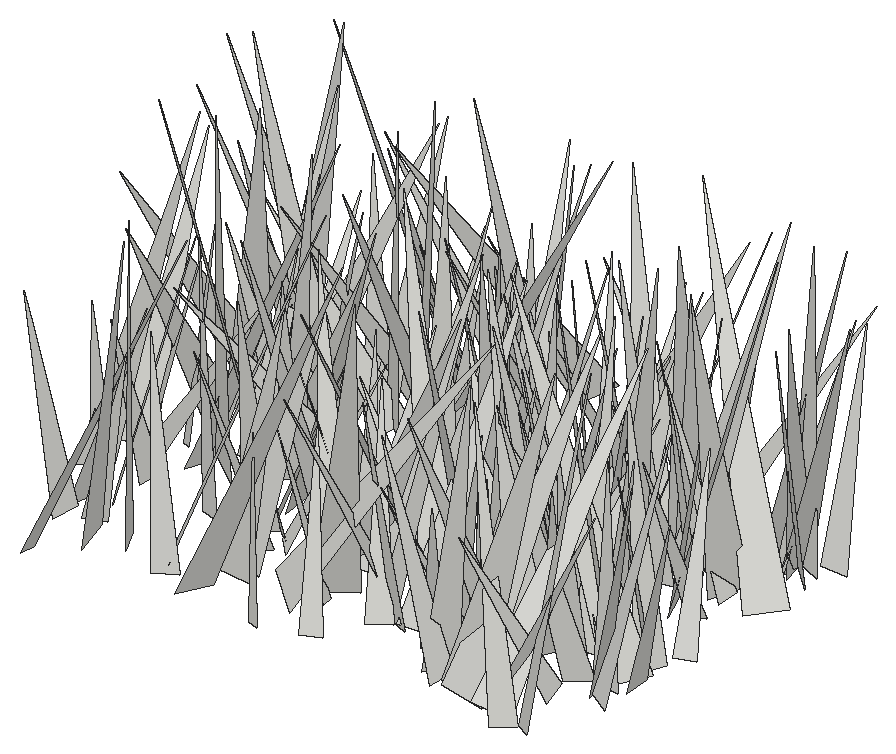
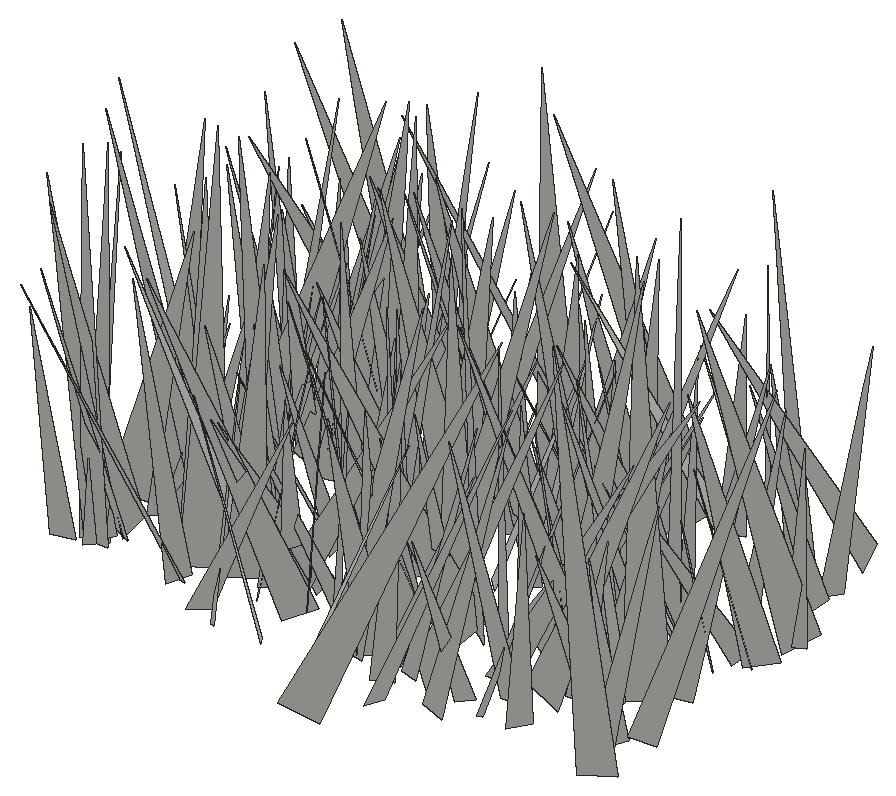
# SketchUp Ruby script. Lengths in inches.
U = 1.inch
M = Sketchup.active_model
def pt(a) = Geom::Point3d.new(a.map { |v| v * U })
def face(e, loops, mat)
  f = e.add_face(loops[0].map { |a| pt(a) })
  loops[1..].each { |l| e.add_face(l.map { |a| pt(a) }).erase! }
  f.material = f.back_material = mat if mat
  f
end
# faces: each face lists its corners as indices into pts; further lists are holes
def faces(e, pts, list, mat = nil) = list.each { |f| face(e, (f[0].is_a?(Array) ? f : [f]).map { |l| l.map { |i| pts[i] } }, mat) }
# xy, xz, yz: faces in a plane at the given z, y or x. An outline is a flat list of corners, or four numbers for a rectangle; further outlines are holes
def ring(l) = l.size == 4 ? [[l[0], l[1]], [l[2], l[1]], [l[2], l[3]], [l[0], l[3]]] : l.each_slice(2).to_a
def flat(e, list, mat, &to3) = list.each { |f| face(e, (f[0].is_a?(Array) ? f : [f]).map { |l| ring(l).map { |u, v| to3.(u, v) } }, mat) }
def xy(e, z, list, mat = nil) = flat(e, list, mat) { |x, y| [x, y, z] }
def xz(e, y, list, mat = nil) = flat(e, list, mat) { |x, z| [x, y, z] }
def yz(e, x, list, mat = nil) = flat(e, list, mat) { |y, z| [x, y, z] }
def lines(e, pts, list) = list.each { |a, b| e.add_line(pt(pts[a]), pt(pts[b])) }
# prism: a flat outline (further loops are holes) pulled along v
def prism(e, loops, v, mat = nil)
  f = face(e, loops, mat); d = Geom::Vector3d.new(v.map { |x| x * U })
  f.pushpull(f.normal.samedirection?(d) ? d.length : -d.length)
end
def box(e, o, s, mat = nil) = prism(e, [[o, [o[0] + s[0], o[1], o[2]], [o[0] + s[0], o[1] + s[1], o[2]], [o[0], o[1] + s[1], o[2]]]], [0, 0, s[2]], mat)
def at(x, y, z, deg = 0) = Geom::Transformation.translation(pt([x, y, z])) * Geom::Transformation.rotation(ORIGIN, Z_AXIS, deg.degrees)
def axes(o, x, y, z) = Geom::Transformation.new([*x, 0, *y, 0, *z, 0, *pt(o).to_a, 1])
def part(name) = M.definitions.add(name)
# library, detail: a bought-in or finely detailed component or shape, given as its bounding box
def library(name, o, s) = part(name).tap { |d| box(d.entities, o, s) }
def detail(e, o, s) = box(e.add_group.entities, o, s)
def put(e, d, t, mat = nil) = e.add_instance(d, t).tap { |i| i.material = mat if mat }
def group(e, t, mat = nil) = e.add_group.tap { |g| g.transformation = t; g.material = mat if mat }.entities
root = M.entities
c1 = part("fur_instance\#9")
p = [[0.8125,0,1.79],[0.67,-0.02,1.48],[0,-0.11,0],[0,0.11,0]]
faces(c1.entities,p,[[0,1,2,3]])
put(root,c1,axes([136.89,288.49,-27.1],[6.91292,1.02767,1.79019],[1.3308,-7.00178,-1.11957],[-1.57792,-1.40299,6.89863]))
put(root,c1,axes([153.03,288.24,-27.1],[-4.85785,0.78834,1.37895],[1.02249,4.94749,0.77364],[1.21552,-1.0112,4.86021]))
put(root,c1,axes([145.31,287.13,-27.1],[1.49909,3.09185,1.25062],[3.12666,-1.78006,0.6529],[-1.16087,-0.8017,3.3735]))
put(root,c1,axes([156.85,289.9,-27.1],[-4.22388,-0.55824,1.0602],[-0.01996,3.91714,1.98304],[1.19803,-1.90295,3.77099]))
put(root,c1,axes([154,288.4,-27.1],[4.37755,-6.1842,1.75356],[-6.40379,-4.01166,1.83857],[0.55746,2.47882,7.3503]))
put(root,c1,axes([140.57,288.07,-27.1],[1.59272,-3.9303,2.28796],[-4.37909,-1.9795,-0.352],[-1.22702,1.96293,4.22612]))
put(root,c1,axes([156.9,286.92,-27.1],[-0.83276,5.81039,0.96307],[5.68734,0.54058,1.65638],[-1.53047,-1.15272,5.63121]))
put(root,c1,axes([142.07,287.86,-27.1],[7.97011,-1.5942,0.50435],[-1.65185,-7.88792,1.1707],[-0.25934,1.24806,8.04323]))
put(root,c1,axes([151.49,289.71,-27.1],[1.84889,-3.8875,0.07331],[-3.87281,-1.83403,0.41727],[0.34554,0.24513,4.2845]))
put(root,c1,axes([152.54,288.78,-27.1],[5.43979,-3.16023,1.66658],[-3.30816,-5.60189,0.17546],[-1.34931,0.9938,6.28869]))
put(root,c1,axes([147.4375,287.77,-27.1],[-1.47,3.64091,0.87512],[3.73843,1.4809,0.11844],[0.21496,-0.85654,3.92467]))
put(root,c1,axes([135.01,289.35,-27.1],[4.20178,-1.75309,2.00996],[-1.5081,-4.65512,-0.90755],[-2.19975,-0.15714,4.46146]))
put(root,c1,axes([146.16,290.82,-27.1],[5.23004,-6.31048,0.45418],[-6.32662,-5.22094,0.31214],[-0.04891,0.54893,8.19012]))
put(root,c1,axes([142.48,289.5,-27.1],[1.87666,-6.19619,1.68038],[-6.32701,-1.4881,1.57887],[1.08876,2.03251,6.27868]))
put(root,c1,axes([155.79,287.94,-27.1],[4.34496,-0.35551,0.43941],[-0.4633,-4.19131,1.19014],[-0.32376,1.22666,4.19388]))
put(root,c1,axes([135.65,286.36,-27.1],[6.20269,2.14266,0.41588],[1.88774,-5.89525,2.21806],[-1.09562,1.97291,6.17613]))
put(root,c1,axes([148.43,291.58,-27.1],[-4.62318,-3.47557,0.41553],[-3.19467,4.47097,1.85217],[1.4305,-1.24775,5.47931]))
put(root,c1,axes([136.17,289.57,-27.1],[2.52401,-3.24586,0.70539],[-3.32076,-2.44552,0.62916],[0.07602,0.94215,4.0633]))
put(root,c1,axes([154.28,289.17,-27.1],[-2.72992,2.63061,1.69887],[2.87463,2.99911,-0.02472],[1.24209,-1.1593,3.79104]))
put(root,c1,axes([154.4,287.71,-27.1],[-0.17327,7.80384,1.95788],[7.72096,0.71202,-2.15474],[2.26272,-1.83203,7.50246]))
put(root,c1,axes([138.12,289.09,-27.1],[5.01686,3.02729,2.73746],[3.17963,-5.61852,0.38618],[-2.55892,-1.04628,5.84673]))
put(root,c1,axes([157.63,287.15,-27.1],[3.93388,5.26717,1.14139],[4.90502,-4.08461,1.94372],[-2.23307,0.30691,6.28017]))
put(root,c1,axes([151.75,291.3125,-27.1],[-3.32799,-2.15223,0.18164],[-2.02775,3.22824,1.09879],[0.74386,-0.82886,3.80792]))
put(root,c1,axes([152.36,292.19,-27.1],[-5.45284,-1.57742,1.94379],[-0.6971,5.43147,2.45217],[2.40429,-2.00271,5.11943]))
put(root,c1,axes([157.73,291.38,-27.1],[5.98567,0.36805,0.66862],[0.55714,-5.71998,-1.83907],[-0.52163,-1.88604,5.70802]))
put(root,c1,axes([144.63,289.7,-27.1],[4.68753,6.76488,0.69054],[6.04009,-3.75687,-4.19721],[3.12373,-2.88717,7.07954]))
put(root,c1,axes([149.41,290.3,-27.1],[1.51862,3.68557,2.40948],[4.21899,-1.94756,0.31991],[-1.2606,-2.07817,3.97332]))
put(root,c1,axes([156.96,291.17,-27.1],[0.96308,-5.75121,1.64983],[-5.7805,-1.32563,-1.24675],[-1.54408,1.37555,5.69645]))
put(root,c1,axes([146.35,290.1,-27.1],[-3.92472,-1.58946,0.29836],[-1.61245,3.78584,-1.04222],[-0.12416,1.07696,4.10409]))
put(root,c1,axes([142.43,290.23,-27.1],[0.67083,5.9533,2.27987],[6.17356,-0.03505,-1.72498],[1.58958,-2.37626,5.73727]))
put(root,c1,axes([134.85,290.2,-27.1],[4.46137,-0.22154,0.62784],[-0.29219,-4.4737,0.49769],[-0.59824,0.53291,4.43905]))
put(root,c1,axes([155.87,287.53,-27.1],[-2.00066,7.03095,0.19663],[6.73059,1.97306,-2.06922],[2.04255,0.38513,7.01108]))
put(root,c1,axes([148.82,289.97,-27.1],[-2.21571,3.96483,0.99922],[4.07213,2.24229,0.13245],[0.36886,-0.93805,4.54001]))
put(root,c1,axes([148.38,293.48,-27.1],[-2.55623,-6.61752,0.06611],[-6.61278,2.55692,0.25211],[0.25899,-0.02922,7.08959]))
put(root,c1,axes([154.93,292.28,-27.1],[3.91329,-2.80057,0.16354],[-2.76188,-3.89534,-0.61821],[-0.49189,-0.40864,4.7723]))
put(root,c1,axes([157.97,291.4,-27.1],[0.13174,-4.85064,1.64659],[-5.10405,0.01535,0.4536],[0.43432,1.65178,4.83118]))
put(root,c1,axes([141.33,292.61,-27.1],[3.50702,-4.68842,0.88051],[-4.69288,-3.58696,-0.4079],[-0.85643,0.45629,5.84073]))
put(root,c1,axes([150.86,291.74,-27.1],[4.29298,-1.68508,0.76366],[-1.68331,-4.35833,-0.1541],[-0.76754,0.13347,4.60928]))
put(root,c1,axes([158.81,292.16,-27.1],[4.67229,-0.63233,0.28263],[-0.57173,-4.60903,-0.86025],[-0.39095,-0.81674,4.63574]))
put(root,c1,axes([149.92,293.97,-27.1],[-3.16207,-7.07316,1.24758],[-6.76016,3.39142,2.09364],[2.42619,0.2311,7.45956]))
put(root,c1,axes([140.27,288.49,-27.1],[5.9455,4.2001,0.21568],[4.05072,-5.81939,1.66213],[-1.13095,1.23699,7.08711]))
put(root,c1,axes([158.41,290.45,-27.1],[2.85218,4.71528,1.10181],[4.83661,-2.83604,-0.38317],[-0.23454,-1.14272,5.49745]))
put(root,c1,axes([155.8,292.32,-27.1],[1.04102,-4.92803,1.21287],[-5.07408,-1.03535,0.14838],[-0.10125,1.21771,5.0346]))
put(root,c1,axes([155.33,292.5,-27.1],[-1.95958,-4.83915,1.26512],[-4.97855,2.01787,0.00704],[0.48156,1.1699,5.22085]))
put(root,c1,axes([142.3,291.72,-27.1],[-1.49858,-3.44059,1.04989],[-3.40031,0.98374,-1.62968],[-1.17382,1.54281,3.38047]))
put(root,c1,axes([135.875,293.13,-27.1],[-3.46561,0.71078,2.1355],[1.4755,3.67824,1.17025],[1.69955,-1.74395,3.33859]))
put(root,c1,axes([145.92,291.18,-27.1],[2.97491,-4.25566,3.74848],[-5.0806,-3.88069,-0.37363],[-2.51977,2.80026,5.17891]))
put(root,c1,axes([153.87,292.34,-27.1],[-5.4764,4.5647,2.90915],[5.14181,5.68019,0.76664],[1.69155,-2.48788,7.08799]))
put(root,c1,axes([158.16,293.69,-27.1],[-3.52584,-3.38703,1.52089],[-2.9555,3.82986,1.67745],[2.24724,-0.27722,4.59235]))
put(root,c1,axes([157.79,291.96,-27.1],[-4.59653,-5.39297,2.39685],[-5.86856,4.49796,-1.13384],[0.62378,2.57709,6.99476]))
put(root,c1,axes([158.34,292.31,-27.1],[-5.06971,5.94983,1.91077],[6.22333,4.58369,2.23904],[-0.56711,-2.88838,7.48926]))
put(root,c1,axes([143.96,293.5,-27.1],[-0.89834,-6.55906,1.37521],[-6.65422,0.70817,-0.96916],[-0.7961,1.48213,6.54897]))
put(root,c1,axes([135.64,291.36,-27.1],[4.69542,3.0157,0.91715],[3.05189,-4.76105,0.03053],[-0.78841,-0.46959,5.58037]))
put(root,c1,axes([145.53,292.83,-27.1],[5.33015,-4.46349,0.382],[-4.4244,-5.15196,1.5366],[0.7024,1.41905,6.78027]))
put(root,c1,axes([144.39,294.38,-27.1],[-3.15103,-4.03715,0.66571],[-3.75697,3.18756,1.54769],[1.62077,-0.46003,4.88182]))
put(root,c1,axes([150.16,290.44,-27.1],[-2.57926,6.41675,1.59968],[6.21683,2.93816,-1.76197],[2.25493,-0.76079,6.68751]))
put(root,c1,axes([133.66,293.0625,-27.1],[1.81522,-3.21568,0.8696],[-3.29805,-1.87418,-0.04607],[-0.46866,0.73395,3.69235]))
put(root,c1,axes([157.86,291.68,-27.1],[-3.7674,-0.4134,0.34529],[-0.49063,3.64055,-0.99453],[0.22227,1.02903,3.6572]))
put(root,c1,axes([154.05,293.89,-27.1],[2.81422,-5.9892,1.8303],[-5.99838,-3.15452,-1.09945],[-1.79999,1.14839,6.52546]))
put(root,c1,axes([150.88,294.37,-27.1],[2.46673,-5.38252,0.46134],[-5.39282,-2.42347,0.55987],[0.31917,0.65147,5.89431]))
put(root,c1,axes([139.17,292.38,-27.1],[1.89742,4.59885,2.05217],[4.78177,-2.33318,0.8074],[-1.57969,-1.53878,4.90894]))
put(root,c1,axes([154.875,293.25,-27.1],[-4.89111,-2.11302,1.38613],[-2.21595,5.03778,-0.13961],[1.21481,0.68196,5.3262]))
put(root,c1,axes([142.64,292.28,-27.1],[3.00056,3.161,0.00616],[3.13284,-2.97269,-0.58633],[0.42105,-0.40809,4.31874]))
put(root,c1,axes([151.18,293.05,-27.1],[4.40781,-2.35415,1.32075],[-2.57038,-4.43283,0.67704],[-0.82436,1.23418,4.95101]))
put(root,c1,axes([142.22,292.78,-27.1],[-6.33694,-5.31771,1.42218],[-5.44687,5.74429,-2.79146],[-0.79519,3.03026,7.78734]))
put(root,c1,axes([156.51,293.7,-27.1],[4.13906,-0.88394,1.08396],[-0.87234,-4.27812,-0.15771],[-1.09332,0.06702,4.22946]))
put(root,c1,axes([158.46,293.41,-27.1],[-4.8782,2.33838,1.88669],[2.5546,5.12175,0.25721],[1.58166,-1.06025,5.40358]))
put(root,c1,axes([148.5,293.75,-27.1],[-3.99734,1.08155,0.32432],[1.12476,3.91891,0.79421],[0.09918,-0.85212,4.0642]))
put(root,c1,axes([148.25,291.2,-27.1],[3.95249,6.61953,0.92655],[6.54498,-4.05132,1.02412],[-1.35642,-0.25967,7.64143]))
put(root,c1,axes([146.36,292.8,-27.1],[0.74046,6.81709,2.01452],[6.9144,-0.22063,-1.79488],[1.64984,-2.13492,6.61811]))
put(root,c1,axes([149.95,295.09,-27.1],[-0.40221,-7.56998,1.93164],[-7.73436,0.65878,0.97125],[1.10251,1.85984,7.51818]))
put(root,c1,axes([141.22,293.54,-27.1],[3.86213,1.08614,0.2172],[1.09096,-3.86634,-0.0646],[-0.19154,-0.12107,4.01143]))
put(root,c1,axes([155.62,295.33,-27.1],[-2.21382,-3.77344,0.32599],[-3.76288,2.23425,0.30817],[0.43109,0.1241,4.36404]))
put(root,c1,axes([145.86,292.68,-27.1],[-1.59343,4.55905,1.08338],[4.45907,1.82697,-1.12985],[1.44061,-0.61229,4.69546]))
put(root,c1,axes([152.04,293.18,-27.1],[-4.34264,3.05124,0.46122],[3.07623,4.34339,0.23041],[0.24406,-0.45414,5.3024]))
put(root,c1,axes([155.55,293.49,-27.1],[-0.37721,6.24874,2.25952],[6.16262,-0.51732,2.45945],[-2.4848,-2.23161,5.75674]))
put(root,c1,axes([141.12,295.125,-27.1],[7.51831,-0.309,0.51299],[-0.23256,-7.46002,-1.08516],[-0.55186,-1.06592,7.446]))
put(root,c1,axes([133.64,292.78,-27.1],[6.60662,-2.19065,2.41659],[-2.83754,-6.55209,1.81792],[-1.6085,2.56075,6.71874]))
put(root,c1,axes([137.42,295.32,-27.1],[-3.84702,-6.56229,2.86732],[-6.71624,4.43571,1.14075],[2.48541,1.82909,7.52076]))
put(root,c1,axes([149.05,293.26,-27.1],[2.27452,-5.56414,4.58515],[-6.58849,-3.55674,-1.04785],[-2.92831,3.68058,5.91904]))
put(root,c1,axes([151.23,293.28,-27.1],[4.54007,-1.04122,1.07478],[-1.33062,-4.37982,1.37772],[-0.68465,1.60765,4.44952]))
put(root,c1,axes([155.875,292.99,-27.1],[0.35449,6.1752,1.09899],[6.2119,-0.49795,0.79425],[-0.86782,-1.04187,6.13416]))
put(root,c1,axes([139.6,293.9,-27.1],[2.64561,4.33348,1.24236],[4.47199,-2.70465,-0.08904],[-0.56902,-1.10798,5.07645]))
put(root,c1,axes([144.87,296.27,-27.1],[-3.28468,-3.33783,0.1825],[-3.30088,3.27904,0.56182],[0.52783,-0.26523,4.64915]))
put(root,c1,axes([147.56,294.5,-27.1],[3.87683,-5.48097,2.21285],[-5.90731,-3.50163,1.67625],[0.20355,2.76859,6.50085]))
put(root,c1,axes([139.79,296.24,-27.1],[3.06125,-3.87557,0.82155],[-3.90702,-3.12527,-0.1848],[-0.65588,0.52812,4.93529]))
put(root,c1,axes([140.46,298.4,-27.1],[-5.57045,-1.42182,0.3414],[-1.0257,4.7578,3.07884],[1.04215,-2.91715,4.85512]))
put(root,c1,axes([134.63,298.59,-27.1],[5.34512,-3.23236,0.64666],[-2.65449,-4.95104,-2.80671],[-1.95449,-2.11559,5.5804]))
put(root,c1,axes([152.01,294.16,-27.1],[-4.80614,1.67739,0.07303],[1.63862,4.73444,-0.90443],[0.36591,0.83033,5.00945]))
put(root,c1,axes([134.17,295.01,-27.1],[2.95956,2.83712,0.75066],[2.89518,-2.997,-0.08741],[-0.48027,-0.58351,4.09885]))
put(root,c1,axes([158.93,294.74,-27.1],[-1.59242,3.59476,0.56652],[3.61736,1.63113,-0.18207],[0.39739,-0.44291,3.92746]))
put(root,c1,axes([143.74,295.6,-27.1],[-2.47,2.58512,1.49197],[2.74392,2.72878,-0.18549],[1.17462,-0.93843,3.57063]))
put(root,c1,axes([134.64,294.88,-27.1],[3.53802,-1.77872,0.68161],[-1.86523,-2.94336,2.00089],[0.38644,2.07817,3.41729]))
put(root,c1,axes([157.32,297.41,-27.1],[0.58704,-3.79537,0.45103],[-3.78334,-0.64184,-0.47675],[-0.5428,0.36891,3.81079]))
put(root,c1,axes([133.78,294.82,-27.1],[-3.09006,5.24053,1.65653],[5.13422,3.43055,-1.27548],[1.9614,-0.72379,5.94851]))
put(root,c1,axes([150.25,297.36,-27.1],[0.10364,-5.95888,1.80759],[-6.13378,0.21397,1.05707],[1.07352,1.79787,5.86529]))
put(root,c1,axes([144.56,299.78,-27.1],[-0.28609,-7.90952,0.17476],[-7.91116,0.28452,-0.07401],[-0.06767,0.17732,7.91434]))
put(root,c1,axes([136.5,294.93,-27.1],[6.82155,0.82248,0.97272],[0.53436,-6.65794,1.88216],[-1.15634,1.77527,6.60814]))
put(root,c1,axes([149.42,296.24,-27.1],[-4.67336,-1.61213,2.14084],[-2.03116,4.93814,-0.71533],[1.7483,1.42769,4.89159]))
put(root,c1,axes([153.91,297.68,-27.1],[6.97924,-1.80721,1.76653],[-1.77915,-7.19853,-0.33521],[-1.79479,0.10824,7.20163]))
put(root,c1,axes([138.93,297.33,-27.1],[6.1687,-0.67373,2.21616],[-0.70194,-6.55164,-0.0379],[-2.20738,0.2006,6.20527]))
put(root,c1,axes([147.09,299.61,-27.1],[-3.51133,-6.12863,1.17286],[-5.90116,3.69891,1.66117],[2.0278,0.152,6.86513]))
put(root,c1,axes([135.3,295.87,-27.1],[2.28996,3.33239,0.84649],[3.03653,-2.43723,1.38011],[-1.61271,0.14282,3.80053]))
put(root,c1,axes([135.39,299.39,-27.1],[5.72891,-5.77899,0.7373],[-5.79412,-5.75966,-0.12335],[-0.60698,0.43635,8.13646]))
put(root,c1,axes([136.48,295.88,-27.1],[3.1839,3.43631,0.24845],[3.39454,-3.18669,0.57383],[-0.5891,0.20968,4.64932]))
put(root,c1,axes([157.11,299.53,-27.1],[6.05759,-4.04132,1.47541],[-3.82561,-6.22554,-1.34569],[-1.96821,-0.33746,7.15653]))
put(root,c1,axes([156.08,297.77,-27.1],[7.78659,2.72532,1.24866],[2.87625,-7.77148,-0.97412],[-0.84485,-1.33952,8.19204]))
put(root,c1,axes([137.41,299.1,-27.1],[2.70621,-3.86796,1.26709],[-3.69816,-2.97221,-1.17466],[-1.70008,0.30833,4.57219]))
put(root,c1,axes([155.84,298,-27.1],[5.68987,2.39384,1.65752],[2.61602,-5.80047,-0.60296],[-1.2784,-1.21517,6.14342]))
put(root,c1,axes([151.81,297.12,-27.1],[1.90499,3.12749,0.05078],[3.06447,-1.8542,-0.76405],[0.62675,-0.43991,3.5814]))
put(root,c1,axes([144.82,298.29,-27.1],[-1.49682,6.02983,3.22428],[6.74332,1.8484,-0.32627],[1.1325,-3.03643,6.20426]))
put(root,c1,axes([133.65,301.79,-27.1],[5.96418,-2.86813,1.57613],[-1.66285,-5.47776,-3.67572],[-2.81874,-2.83722,5.50334]))
put(root,c1,axes([154.67,298.51,-27.1],[-0.07394,-6.12578,2.47714],[-6.56947,-0.19789,-0.68546],[-0.70961,2.47033,6.08776]))
put(root,c1,axes([156.03,298.87,-27.1],[-1.67476,-3.89018,1.26522],[-4.03938,1.78862,0.15259],[0.64624,1.09838,4.23261]))
put(root,c1,axes([137.97,298.65,-27.1],[3.87779,-2.1954,0.31482],[-2.2129,-3.78759,0.8446],[0.14815,0.88911,4.37535]))
put(root,c1,axes([141.53,298.27,-27.1],[-3.36679,-6.63148,1.92496],[-6.20382,1.96447,-4.08298],[-3.03226,3.34389,6.21619]))
put(root,c1,axes([150.87,297.67,-27.1],[4.041,0.55824,1.1889],[0.26805,-4.11576,1.02147],[-1.28579,0.89645,3.94942]))
put(root,c1,axes([143,299.46,-27.1],[-4.52397,-6.09316,3.51067],[-6.34353,5.33763,1.08955],[3.03497,2.07386,7.51038]))
put(root,c1,axes([157.33,299.18,-27.1],[-4.29082,0.07848,0.62907],[0.12494,4.3243,0.31276],[0.62151,-0.32753,4.28013]))
put(root,c1,axes([139.02,299.63,-27.1],[-7.80525,1.8691,2.4402],[2.24771,8.01322,1.05174],[2.09664,-1.63243,7.95672]))
put(root,c1,axes([149.01,298.01,-27.1],[-2.72966,-3.54913,3.67888],[-4.47058,3.67982,0.23296],[2.47878,2.72838,4.47136]))
put(root,c1,axes([147.49,297.79,-27.1],[-3.18847,2.06393,0.29466],[1.98964,3.17316,-0.69666],[0.62286,0.42918,3.73374]))
put(root,c1,axes([150.45,300.67,-27.1],[-1.24481,-6.10899,0.55091],[-5.80958,0.99391,-2.10566],[-1.96776,0.93016,5.86818]))
put(root,c1,axes([137.82,296.35,-27.1],[1.84381,6.83005,0.32521],[6.75707,-1.87158,0.99709],[-1.04756,-0.05069,7.00393]))
put(root,c1,axes([135.87,300.07,-27.1],[5.69454,1.71793,1.14191],[1.95584,-5.5622,-1.38552],[-0.6557,-1.67144,5.78441]))
put(root,c1,axes([145.58,300.45,-27.1],[5.69502,0.05498,1.49404],[0.36012,-5.7612,-1.16071],[-1.45103,-1.21405,5.57575]))
put(root,c1,axes([153.75,301.67,-27.1],[4.25947,-6.86655,0.67935],[-6.89421,-4.26807,0.08653],[-0.2843,0.62304,8.07992]))
put(root,c1,axes([154.02,301.58,-27.1],[3.44417,-6.15496,0.43731],[-6.17002,-3.42915,0.33004],[0.07525,0.54268,7.04535]))
put(root,c1,axes([146.01,297.75,-27.1],[2.63979,2.66437,0.28601],[2.37928,-2.51517,1.47039],[-1.23275,0.85099,3.4504]))
put(root,c1,axes([158.18,302.22,-27.1],[-3.37811,-5.89928,1.5704],[-5.1932,3.72048,2.80499],[3.2091,-0.18922,6.19235]))
put(root,c1,axes([155.06,299.52,-27.1],[-0.81294,-7.33898,4.00432],[-7.82592,2.08335,2.22952],[2.94113,3.51498,7.03923]))
put(root,c1,axes([144.15,299.39,-27.1],[3.92282,-1.4058,1.44453],[-1.66907,-4.03753,0.60333],[-1.1301,1.0833,4.1232]))
put(root,c1,axes([151.07,301.35,-27.1],[3.64038,-1.44849,0.64201],[-1.22649,-3.59476,-1.15586],[-1.003,-0.8615,3.74359]))
put(root,c1,axes([151.11,300.17,-27.1],[4.61454,1.12705,1.27743],[1.23829,-4.75228,-0.2803],[-1.16993,-0.58453,4.7419]))
put(root,c1,axes([139.31,303.99,-27.1],[-5.60645,-3.595,0.79099],[-2.74257,5.04084,3.47133],[2.4552,-2.57833,5.68385]))
put(root,c1,axes([157.8,302.71,-27.1],[7.1612,-0.61813,1.17268],[-0.1707,-6.81898,-2.55193],[-1.31459,-2.48182,6.71956]))
put(root,c1,axes([137.47,300.91,-27.1],[3.73633,3.15118,1.53756],[3.50493,-3.41917,-1.50964],[-0.09758,-2.15258,4.64878]))
put(root,c1,axes([140.33,301.53,-27.1],[-4.08347,2.98679,1.40676],[3.27171,3.36098,2.36101],[-0.44252,-2.71247,4.47451]))
put(root,c1,axes([145.95,299.3,-27.1],[0.78964,4.34465,0.57519],[4.335,-0.86018,0.54605],[-0.64386,-0.46311,4.38193]))
put(root,c1,axes([145.29,302.74,-27.1],[4.67947,-2.49587,0.44393],[-2.29207,-4.56374,-1.49753],[-1.08298,-1.12554,5.08765]))
put(root,c1,axes([136.49,300.46,-27.1],[1.93796,6.92662,2.2466],[6.80944,-0.90011,-3.09877],[2.58009,-2.82714,6.49087]))
put(root,c1,axes([151.92,300.3,-27.1],[-1.54169,4.36128,2.00643],[4.43238,2.10262,-1.16464],[1.84406,-1.40768,4.47674]))
put(root,c1,axes([147.75,301.64,-27.1],[-1.86728,-3.21645,1.13397],[-3.16749,2.11482,0.78275],[1.26429,0.54787,3.63587]))
put(root,c1,axes([143.25,299.49,-27.1],[7.82793,-0.68601,0.13891],[-0.69946,-7.6099,1.83483],[0.02566,1.8399,7.64072]))
put(root,c1,axes([159.06,299.24,-27.1],[-3.56857,7.17935,0.49748],[7.02506,3.35468,1.97986],[-1.56176,-1.31463,7.76903]))
put(root,c1,axes([140.17,301.51,-27.1],[-3.26006,-5.04679,2.60885],[-5.29814,3.78652,0.70434],[2.05082,1.75965,5.96674]))
put(root,c1,axes([149.16,301.51,-27.1],[-3.54566,-2.66431,1.6705],[-2.78653,3.82874,0.19209],[1.45754,0.83849,4.43096]))
put(root,c1,axes([157.85,302.4,-27.1],[6.64533,-1.36705,0.39109],[-1.31179,-6.61549,-0.83466],[-0.54862,-0.74069,6.73295]))
put(root,c1,axes([148.16,300.91,-27.1],[1.07989,-3.22676,1.49499],[-3.22529,-0.23045,1.83235],[1.49815,1.82977,2.86716]))
put(root,c1,axes([138.46,301.5,-27.1],[-0.67807,6.71445,3.30984],[6.96597,-0.65101,2.74773],[-2.74118,-3.31527,6.16389]))
put(root,c1,axes([146.5,298.57,-27.1],[4.01654,5.38759,0.39242],[5.219,-3.99648,1.45013],[-1.3936,0.56102,6.56169]))
put(root,c1,axes([149.51,300.05,-27.1],[3.96425,-0.56902,0.64503],[-0.79665,-3.57598,1.74151],[-0.32433,1.82859,3.60641]))
put(root,c1,axes([144.28,302.75,-27.1],[-0.56318,-3.80765,0.20803],[-3.75255,0.51599,-0.71463],[-0.67806,0.30692,3.78215]))
put(root,c1,axes([151.1,301.88,-27.1],[-4.28874,-2.62611,1.19653],[-2.76089,4.3576,-0.33198],[0.84,0.91449,5.01792]))
put(root,c1,axes([143.14,303.27,-27.1],[-1.82356,-4.42835,0.39133],[-4.41286,1.85435,0.42054],[0.53859,0.19978,4.77062]))
put(root,c1,axes([157.94,302.7,-27.1],[-1.4348,-7.0433,2.45033],[-7.23254,1.92235,1.29061],[1.81726,2.08982,7.07114]))
put(root,c1,axes([137.26,300.93,-27.1],[-1.4583,4.1794,0.64732],[4.14586,1.27741,1.09233],[-0.83566,-0.95598,4.28962]))
put(root,c1,axes([152.375,300.47,-27.1],[6.025,3.41302,0.55167],[3.40656,-6.04972,0.22351],[-0.59027,-0.07668,6.92094]))
put(root,c1,axes([150.62,300.47,-27.1],[-4.55116,2.07867,0.64916],[1.93391,4.54938,-1.00919],[1.00113,0.66152,4.90056]))
put(root,c1,axes([152.11,301.375,-27.1],[-4.3858,5.26104,2.02142],[5.54364,4.48874,0.34523],[1.01623,-1.78118,6.84066]))
put(root,c1,axes([157.5,300.99,-27.1],[6.67173,1.075,1.66778],[0.88806,-6.84957,0.86244],[-1.77439,0.61387,6.70252]))
put(root,c1,axes([151.73,299.41,-27.1],[-3.94545,3.07895,0.18102],[2.74281,3.63702,-2.08047],[1.41057,1.53994,4.55172]))
put(root,c1,axes([146.3125,302.24,-27.1],[-4.08433,-4.26667,3.28401],[-4.58243,4.91876,0.69141],[2.82675,1.80893,5.86585]))
put(root,c1,axes([147.05,301.52,-27.1],[0.66208,3.60921,1.19442],[3.54519,-1.02396,1.12897],[-1.37285,-0.90361,3.49144]))
put(root,c1,axes([153.87,302.93,-27.1],[5.53978,-0.90724,0.62547],[-0.85463,-5.56113,-0.49688],[-0.69563,-0.39269,5.59154]))
put(root,c1,axes([143.62,304.14,-27.1],[0.2783,-5.0487,0.14304],[-4.93686,-0.24166,1.07529],[1.0664,0.19877,4.94071]))
put(root,c1,axes([134.23,303.51,-27.1],[-0.19346,-4.85951,0.89963],[-4.92735,0.1202,-0.41034],[-0.38132,0.91231,4.84602]))
put(root,c1,axes([157.51,301.65,-27.1],[2.91311,4.64162,1.0633],[4.76072,-2.81168,-0.76908],[0.10392,-1.30816,5.4258]))
put(root,c1,axes([134.22,302.44,-27.1],[3.08181,-1.73974,0.98019],[-1.88437,-3.1302,0.36886],[-0.66077,0.81254,3.51969]))
put(root,c1,axes([136.17,301.27,-27.1],[-2.24412,3.20659,0.81725],[3.00578,2.38826,-1.11699],[1.38398,0.01256,3.75108]))
put(root,c1,axes([146.07,303.26,-27.1],[-0.62718,-6.98929,2.39617],[-7.29856,0.2117,-1.29283],[-1.15016,2.46782,6.89725]))
put(root,c1,axes([148.93,302.21,-27.1],[3.61026,-5.57217,1.81458],[-5.57053,-2.60139,3.09478],[1.81959,3.09184,5.87413]))
put(root,c1,axes([145.1,302.92,-27.1],[-2.61332,3.50076,2.27341],[3.90248,3.00092,-0.13507],[1.48133,-1.72983,4.36652]))
put(root,c1,axes([142.74,303,-27.1],[-5.1387,-6.17044,1.38685],[-6.22365,4.61615,-2.52214],[-1.12419,2.64967,7.62361]))
put(root,c1,axes([150.91,304.73,-27.1],[-2.708,-3.38854,1.07596],[-2.8715,2.88211,1.84961],[2.09627,-0.42942,3.92357]))
put(root,c1,axes([140.82,304.8,-27.1],[-1.81224,-5.34948,0.90018],[-5.42401,1.80193,-0.21131],[0.08596,0.92064,5.64415]))
put(root,c1,axes([133.36,304.75,-27.1],[1.45469,-7.67033,1.86376],[-7.74266,-1.0178,1.85445],[1.53584,2.13396,7.5836]))
put(root,c1,axes([139,302.49,-27.1],[0.94432,5.62245,1.27282],[5.76049,-0.87093,-0.42662],[0.22085,-1.32412,5.68522]))
put(root,c1,axes([153.79,302.94,-27.1],[3.84668,4.92623,0.09388],[4.62666,-3.57049,-2.21792],[1.69428,-1.43435,5.84342]))
put(root,c1,axes([159.04,303.08,-27.1],[-0.27729,4.76979,1.49646],[4.98187,0.38774,-0.31274],[0.41383,-1.47171,4.7676]))
put(root,c1,axes([142.85,305.59,-27.1],[-6.28485,-0.79991,0.77187],[-0.56549,6.11624,1.73401],[0.95701,-1.63912,6.09364]))
put(root,c1,axes([144.49,307.82,-27.1],[4.16443,-6.48584,0.7003],[-5.50995,-3.94185,-3.74183],[-3.49241,-1.51483,6.7385]))
put(root,c1,axes([137.76,303.66,-27.1],[3.42061,-2.16163,2.16053],[-2.46149,-3.8706,0.02453],[-1.81151,1.17767,4.04631]))
put(root,c1,axes([152,304.12,-27.1],[-4.37284,2.10544,0.41102],[2.13916,4.20984,1.19366],[-0.16073,-1.25217,4.70423]))
put(root,c1,axes([145.84,301.89,-27.1],[-5.09281,3.29268,0.78292],[3.01884,5.05892,-1.63872],[1.53013,0.9783,5.83893]))
put(root,c1,axes([145.91,306.07,-27.1],[-3.80651,-3.12707,0.03174],[-3.06593,3.74155,0.93273],[0.61617,-0.70095,4.83716]))
put(root,c1,axes([148.8,304.57,-27.1],[3.81482,2.67004,0.71919],[2.75746,-3.58156,-1.32965],[0.20681,-1.49748,4.4625]))
put(root,c1,axes([140.4,303.45,-27.1],[-1.29453,3.3269,0.92168],[3.25121,1.50588,-0.8692],[1.16077,-0.50757,3.46245]))
